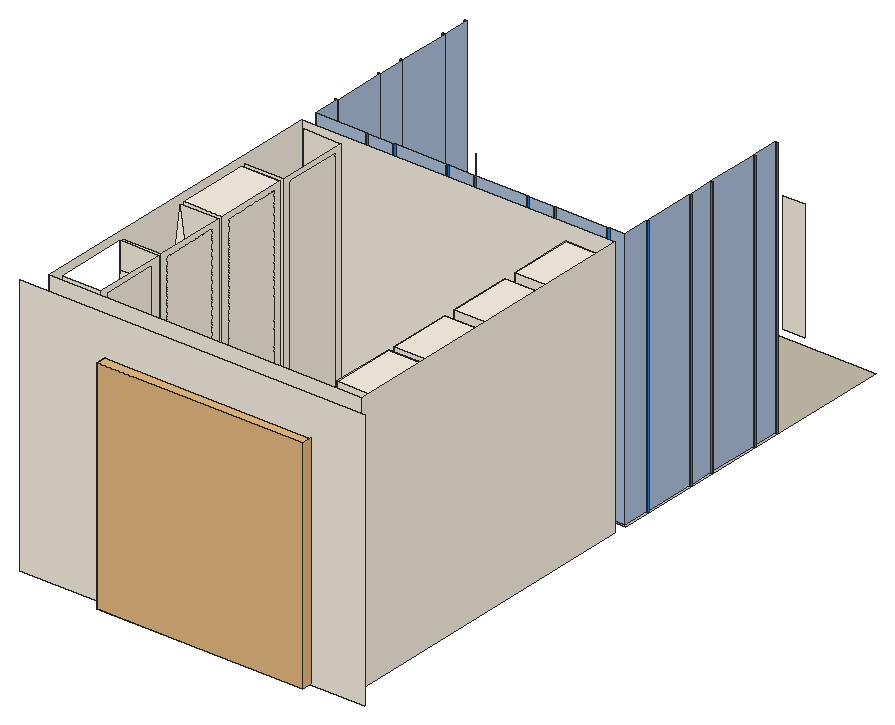
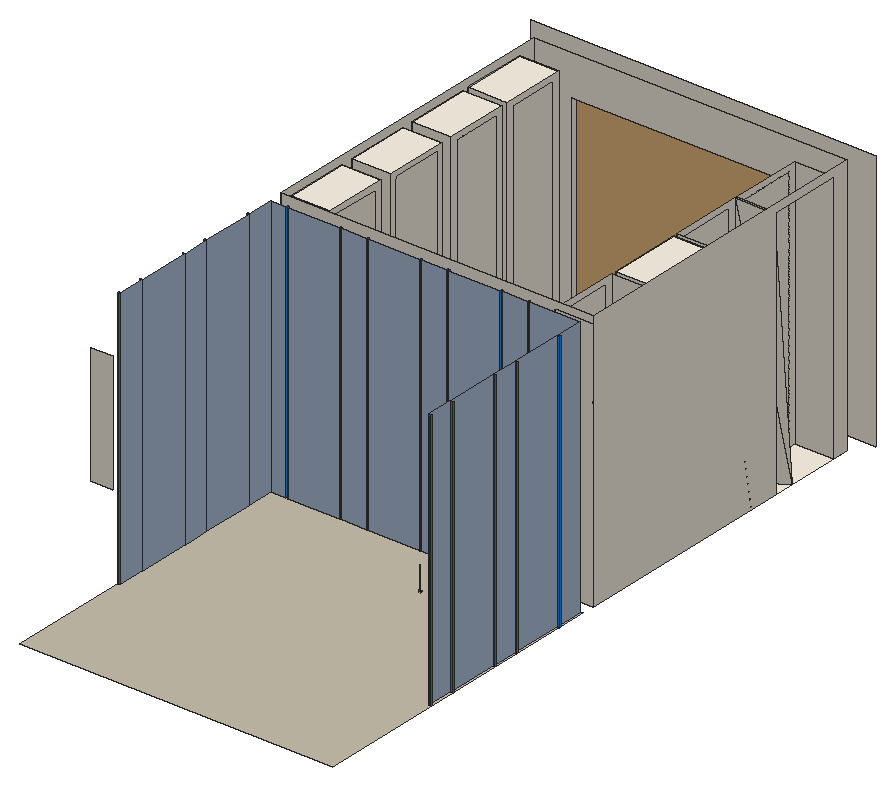
# SketchUp Ruby script. Lengths in inches.
U = 1.inch
M = Sketchup.active_model
def pt(a) = Geom::Point3d.new(a.map { |v| v * U })
def face(e, loops, mat)
  f = e.add_face(loops[0].map { |a| pt(a) })
  loops[1..].each { |l| e.add_face(l.map { |a| pt(a) }).erase! }
  f.material = f.back_material = mat if mat
  f
end
# faces: each face lists its corners as indices into pts; further lists are holes
def faces(e, pts, list, mat = nil) = list.each { |f| face(e, (f[0].is_a?(Array) ? f : [f]).map { |l| l.map { |i| pts[i] } }, mat) }
# xy, xz, yz: faces in a plane at the given z, y or x. An outline is a flat list of corners, or four numbers for a rectangle; further outlines are holes
def ring(l) = l.size == 4 ? [[l[0], l[1]], [l[2], l[1]], [l[2], l[3]], [l[0], l[3]]] : l.each_slice(2).to_a
def flat(e, list, mat, &to3) = list.each { |f| face(e, (f[0].is_a?(Array) ? f : [f]).map { |l| ring(l).map { |u, v| to3.(u, v) } }, mat) }
def xy(e, z, list, mat = nil) = flat(e, list, mat) { |x, y| [x, y, z] }
def xz(e, y, list, mat = nil) = flat(e, list, mat) { |x, z| [x, y, z] }
def yz(e, x, list, mat = nil) = flat(e, list, mat) { |y, z| [x, y, z] }
def lines(e, pts, list) = list.each { |a, b| e.add_line(pt(pts[a]), pt(pts[b])) }
# prism: a flat outline (further loops are holes) pulled along v
def prism(e, loops, v, mat = nil)
  f = face(e, loops, mat); d = Geom::Vector3d.new(v.map { |x| x * U })
  f.pushpull(f.normal.samedirection?(d) ? d.length : -d.length)
end
def box(e, o, s, mat = nil) = prism(e, [[o, [o[0] + s[0], o[1], o[2]], [o[0] + s[0], o[1] + s[1], o[2]], [o[0], o[1] + s[1], o[2]]]], [0, 0, s[2]], mat)
def at(x, y, z, deg = 0) = Geom::Transformation.translation(pt([x, y, z])) * Geom::Transformation.rotation(ORIGIN, Z_AXIS, deg.degrees)
def axes(o, x, y, z) = Geom::Transformation.new([*x, 0, *y, 0, *z, 0, *pt(o).to_a, 1])
def part(name) = M.definitions.add(name)
# library, detail: a bought-in or finely detailed component or shape, given as its bounding box
def library(name, o, s) = part(name).tap { |d| box(d.entities, o, s) }
def detail(e, o, s) = box(e.add_group.entities, o, s)
def put(e, d, t, mat = nil) = e.add_instance(d, t).tap { |i| i.material = mat if mat }
def group(e, t, mat = nil) = e.add_group.tap { |g| g.transformation = t; g.material = mat if mat }.entities
root = M.entities
M.materials.add("Material \#1").color = [140, 140, 140]
M.materials.add("[0030_OldLace]").color = [253, 245, 230]
M.materials.add("[0098_DodgerBlue]").color = [30, 144, 255]
M.materials.add("[0099_LightSteelBlue]").color = [176, 196, 222]
M.materials.add("[Tile Canvas]").color = [199, 192, 173]
c1 = library("Shutters 03 47-19",[-43.47,-3.54,0],[86.94,7.08,66.14])
xy(root,0,[[392.77,22.3125,410.71,51.82],[392.77,54.66,410.71,84.17],[392.77,89.42,410.71,118.93],[392.77,124.42,410.71,153.93]])
xy(root,116.41,[[392.77,22.3125,410.71,51.82],[392.77,54.66,410.71,84.17],[392.77,89.42,410.71,118.93],[267.03,90.88,284.97,124.24],[392.77,124.42,410.71,153.93]],"[0030_OldLace]")
xz(root,4.46,[[261,0,300.25,0,300.25,101.375,393.62,101.375,393.62,0,420,0,420,120,261,120]],"[0030_OldLace]")
xz(root,13.46,[[267,0,267,120,411,120,411,0,393.62,0,393.62,101.375,300.25,101.375,300.25,0]],"[0030_OldLace]")
xz(root,20.99,[[267,0,284.9375,116.41]],"[0030_OldLace]")
xz(root,22.3125,[[392.77,0,410.71,116.41]],"[0030_OldLace]")
xz(root,51.82,[[392.77,0,410.71,116.41]],"[0030_OldLace]")
xz(root,54.35,[[267,0,284.9375,116.41]],"[0030_OldLace]")
xz(root,54.66,[[392.77,0,410.71,116.41]],"[0030_OldLace]")
xz(root,84.17,[[392.77,0,410.71,116.41]],"[0030_OldLace]")
xz(root,88.74,[[284.97,0,267.03,116.41,284.97,116.41]],"[0030_OldLace]")
xz(root,89.42,[[392.77,0,410.71,116.41]],"[0030_OldLace]")
xz(root,90.88,[[267.03,0,284.97,116.41]],"[0030_OldLace]")
xz(root,118.93,[[392.77,0,410.71,116.41]],"[0030_OldLace]")
xz(root,124.24,[[267.03,0,284.97,116.41]],"[0030_OldLace]")
xz(root,124.42,[[392.77,0,410.71,116.41]],"[0030_OldLace]")
xz(root,126.11,[[267.03,0,284.97,116.41]],"[0030_OldLace]")
xz(root,153.93,[[392.77,0,410.71,116.41]],"[0030_OldLace]")
xz(root,159.46,[[267,0,267.03,0,267.03,116.41,284.97,116.41,284.97,0,411,0,411,120,267,120],[267.03,0,284.97,116.41]],"[0030_OldLace]")
xz(root,165.46,[[291.48,0,292.01,120],[304,0,304.5,120],[328.5,0,329,120],[341,0,341.45,120],[365.49,0,366,120],
  [378.01,0,378.5,120],[402.49,0,403,120]],"[0098_DodgerBlue]")
xz(root,166.15,[[267.8125,0,291.48,120],[292.01,0,304,120],[304.5,0,328.5,120],[329,0,341,120],[341.45,0,365.49,120],
  [366,0,378.01,120],[378.5,0,402.49,120],[403,0,410,120]],"[0099_LightSteelBlue]")
xz(root,178.44,[[410,0,411,120]],"[0098_DodgerBlue]")
xz(root,178.47,[[267,0,267.8125,120]],"[0098_DodgerBlue]")
xz(root,178.96,[[267,0,268.125,120]],"[0098_DodgerBlue]")
xz(root,179,[[410,0,411,120]],"[0098_DodgerBlue]")
xz(root,202.96,[[267,0,268.125,120],[410,0,411,120]],"[0098_DodgerBlue]")
xz(root,203.46,[[267,0,268.125,120],[410,0,411,120]],"[0098_DodgerBlue]")
xz(root,215.46,[[267,0,268.125,120],[410,0,411,120]],"[0098_DodgerBlue]")
xz(root,215.96,[[267,0,268.125,120],[410,0,411,120]],"[0098_DodgerBlue]")
xz(root,239.96,[[267,0,268.125,120]],"[0098_DodgerBlue]")
xz(root,239.97,[[410,0,411,120]],"[0098_DodgerBlue]")
xz(root,240.46,[[267,0,268.125,120]],"[0098_DodgerBlue]")
xz(root,240.47,[[410,0,411,120]],"[0098_DodgerBlue]")
xz(root,252.47,[[410,0,411,120]],"[0098_DodgerBlue]")
xz(root,252.53,[[267,0,268.125,120]],"[0098_DodgerBlue]")
xz(root,252.96,[[410,0,411,120]],"[0098_DodgerBlue]")
xz(root,253,[[267,0,268.125,120]],"[0098_DodgerBlue]")
xz(root,257.09,[[410,41,420,96]],"[0030_OldLace]")
yz(root,265.64,[[260.51,50.65,260.4,50.66,260.4,50.68],[260.4,50.66,260.29,50.7,260.29,50.72],[260.4,50.66,260.29,50.72,260.4,50.68],[260.29,50.7,260.18,50.77,260.19,50.78],[260.29,50.7,260.19,50.78,260.29,50.72],
  [260.18,50.77,260.09,50.85,260.1,50.86],[260.18,50.77,260.1,50.86,260.19,50.78],[260.09,50.85,260.02,50.95,260.02,50.96],[260.09,50.85,260.02,50.96,260.1,50.86],[260.48,50.88,260.4375,50.9,260.44,50.91],
  [260.48,50.88,260.44,50.91,260.48,50.9],[260.4375,50.9,260.4,50.92,260.41,50.93],[260.4375,50.9,260.41,50.93,260.44,50.91],[260.4,50.92,260.375,50.95,260.38,50.96],[260.4,50.92,260.38,50.96,260.41,50.93],
  [260.02,50.95,259.96,51.08,260.02,50.96],[260.375,50.95,260.35,50.98,260.36,50.99],[260.375,50.95,260.36,50.99,260.38,50.96],[260.35,50.98,260.33,51.02,260.34,51.03],[260.35,50.98,260.34,51.03,260.36,50.99],
  [260.33,51.02,260.3125,51.07,260.32,51.07],[260.33,51.02,260.32,51.07,260.34,51.03],[260.3125,51.07,260.3,51.12,260.3125,51.12],[260.3125,51.07,260.3125,51.12,260.32,51.07],[260.3,51.12,260.3,51.15,260.31,51.15],
  [260.3,51.12,260.31,51.15,260.3125,51.12],[260.3,51.15,260.3,51.22,260.3125,51.22],[260.3,51.15,260.3125,51.22,260.31,51.15],[260.3,51.22,260.3125,51.27,260.32,51.26],[260.3,51.22,260.32,51.26,260.3125,51.22],
  [260.32,51.26,260.3125,51.27,260.34,51.31],[260.3125,51.27,260.33,51.3125,260.34,51.31],[260.34,51.31,260.33,51.3125,260.36,51.34],[260.33,51.3125,260.35,51.35,260.36,51.34],[260.36,51.34,260.35,51.35,260.38,51.375],
  [260.35,51.35,260.375,51.39,260.38,51.375],[260.38,51.375,260.375,51.39,260.41,51.4],[260.375,51.39,260.4,51.42,260.41,51.4],[260.41,51.4,260.4,51.42,260.44,51.42],[260.4,51.42,260.4375,51.4375,260.44,51.42],
  [260.44,51.42,260.4375,51.4375,260.48,51.4375],[260.4375,51.4375,260.48,51.45,260.48,51.4375]],"Material \#1")
yz(root,266.47,[[260.51,50.65,260.4,50.68,260.4,50.66],[260.4,50.66,260.29,50.72,260.29,50.7],[260.4,50.66,260.4,50.68,260.29,50.72],[260.29,50.7,260.19,50.78,260.18,50.77],[260.29,50.7,260.29,50.72,260.19,50.78],
  [260.18,50.77,260.1,50.86,260.09,50.85],[260.18,50.77,260.19,50.78,260.1,50.86],[260.09,50.85,260.02,50.96,260.02,50.95],[260.09,50.85,260.1,50.86,260.02,50.96],[260.48,50.88,260.44,50.91,260.4375,50.9],
  [260.48,50.88,260.48,50.9,260.44,50.91],[260.4375,50.9,260.41,50.93,260.4,50.92],[260.4375,50.9,260.44,50.91,260.41,50.93],[260.4,50.92,260.38,50.96,260.375,50.95],[260.4,50.92,260.41,50.93,260.38,50.96],
  [260.02,50.95,259.96,51.08,259.95,51.08],[260.02,50.95,260.02,50.96,259.96,51.08],[260.375,50.95,260.36,50.99,260.35,50.98],[260.375,50.95,260.38,50.96,260.36,50.99],[260.35,50.98,260.34,51.03,260.33,51.02],
  [260.35,50.98,260.36,50.99,260.34,51.03],[260.33,51.02,260.32,51.07,260.3125,51.07],[260.33,51.02,260.34,51.03,260.32,51.07],[260.3125,51.07,260.3125,51.12,260.3,51.12],[260.3125,51.07,260.32,51.07,260.3125,51.12],
  [259.95,51.08,259.91,51.22,259.9,51.21],[259.95,51.08,259.96,51.08,259.91,51.22],[260.3,51.12,260.31,51.15,260.3,51.15],[260.3,51.12,260.3125,51.12,260.31,51.15],[260.3,51.15,260.31,51.15,260.3125,51.22],
  [260.3,51.15,260.3125,51.22,260.3,51.22],[259.9,51.21,259.88,51.36,259.87,51.36],[259.9,51.21,259.91,51.22,259.88,51.36],[260.3,51.22,260.3125,51.22,260.32,51.26],[260.3,51.22,260.32,51.26,260.3125,51.27],
  [260.32,51.26,260.34,51.31,260.3125,51.27],[260.3125,51.27,260.34,51.31,260.33,51.3125],[260.34,51.31,260.36,51.34,260.33,51.3125],[260.33,51.3125,260.36,51.34,260.35,51.35],[260.36,51.34,260.38,51.375,260.35,51.35],
  [260.35,51.35,260.38,51.375,260.375,51.39],[259.87,51.36,259.87,51.52,259.86,51.52],[259.87,51.36,259.88,51.36,259.87,51.52],[260.38,51.375,260.41,51.4,260.375,51.39],[260.375,51.39,260.41,51.4,260.4,51.42],
  [260.41,51.4,260.44,51.42,260.4,51.42],[260.4,51.42,260.44,51.42,260.4375,51.4375],[260.44,51.42,260.48,51.4375,260.4375,51.4375],[260.4375,51.4375,260.48,51.4375,260.48,51.45],[259.86,51.52,259.87,51.52,259.87,61.41],
  [259.86,51.52,259.87,61.41,259.86,61.42]],"Material \#1")
yz(root,267,[[13.46,0,20.99,0,20.99,116.41,54.35,116.41,54.35,0,159.46,0,159.46,120,13.46,120]],"[0030_OldLace]")
yz(root,267,[[178.47,0,178.96,120],[202.96,0,203.46,120],[215.46,0,215.96,120],[239.96,0,240.46,120],[252.53,0,253,120]],"[0098_DodgerBlue]")
yz(root,267.8125,[[166.15,0,178.47,120]],"[0099_LightSteelBlue]")
yz(root,268.125,[[178.96,0,202.96,120],[203.46,0,215.46,120],[215.96,0,239.96,120],[240.46,0,252.53,120]],"[0099_LightSteelBlue]")
yz(root,284.9375,[[[20.99,0,54.35,116.41],[24.58,2.54,50.75,113.87]],[24.58,2.54,50.75,113.87]],"[0030_OldLace]")
yz(root,284.97,[[[55.39,0,88.74,116.41],[58.98,2.54,85.15,113.87]],[[90.88,0,124.24,116.41],[94.47,2.54,120.64,113.87]],[[126.11,0,159.46,116.41],[129.7,2.54,155.875,113.87]],[58.98,2.54,85.15,113.87],[94.47,2.54,120.64,113.87],
  [129.7,2.54,155.875,113.87]],"[0030_OldLace]")
yz(root,291.48,[[165.46,0,166.15,120]],"[0098_DodgerBlue]")
yz(root,292.01,[[165.46,0,166.15,120]],"[0098_DodgerBlue]")
yz(root,300.25,[[4.46,0,13.46,101.375]],"[0030_OldLace]")
yz(root,304,[[165.46,0,166.15,120]],"[0098_DodgerBlue]")
yz(root,304.5,[[165.46,0,166.15,120]],"[0098_DodgerBlue]")
yz(root,328.5,[[165.46,0,166.15,120]],"[0098_DodgerBlue]")
yz(root,329,[[165.46,0,166.15,120]],"[0098_DodgerBlue]")
yz(root,341,[[165.46,0,166.15,120]],"[0098_DodgerBlue]")
yz(root,341.45,[[165.46,0,166.15,120]],"[0098_DodgerBlue]")
yz(root,365.49,[[165.46,0,166.15,120]],"[0098_DodgerBlue]")
yz(root,366,[[165.46,0,166.15,120]],"[0098_DodgerBlue]")
yz(root,378.01,[[165.46,0,166.15,120]],"[0098_DodgerBlue]")
yz(root,378.5,[[165.46,0,166.15,120]],"[0098_DodgerBlue]")
yz(root,392.77,[[[22.3125,0,51.82,116.41],[25.49,2.54,48.65,113.87]],[[54.66,0,84.17,116.41],[57.83,2.54,80.99,113.87]],[[89.42,0,118.93,116.41],[92.6,2.54,115.76,113.87]],[[124.42,0,153.93,116.41],[127.6,2.54,150.76,113.87]],[25.49,2.54,48.65,113.87],
  [57.83,2.54,80.99,113.87],[92.6,2.54,115.76,113.87],[127.6,2.54,150.76,113.87]],"[0030_OldLace]")
yz(root,393.62,[[4.46,0,13.46,101.375]],"[0030_OldLace]")
yz(root,402.49,[[165.46,0,166.15,120]],"[0098_DodgerBlue]")
yz(root,403,[[165.46,0,166.15,120]],"[0098_DodgerBlue]")
yz(root,410,[[166.15,0,178.44,120],[179,0,202.96,120],[203.46,0,215.46,120],[215.96,0,239.97,120],[240.47,0,252.47,120]],"[0099_LightSteelBlue]")
yz(root,410.71,[[22.3125,0,51.82,116.41],[54.66,0,84.17,116.41],[89.42,0,118.93,116.41],[124.42,0,153.93,116.41]])
yz(root,411,[[13.46,0,159.46,120]],"[0030_OldLace]")
yz(root,411,[[178.44,0,179,120],[202.96,0,203.46,120],[215.46,0,215.96,120],[239.97,0,240.47,120],[252.47,0,252.96,120]],"[0098_DodgerBlue]")
p = [[267.03,55.39,116.41],[267.03,45.34,0],[284.97,55.39,116.41],[284.97,55.39,0],[283.11,54.35,0],[267.03,68.95,0],
  [267.03,88.74,116.41],[284.97,88.74,0],[300.25,13.46,0],[393.62,13.46,0]]
faces(root,p,[[0,1,2],[3,2,1,4],[5,6,7]],"[0030_OldLace]")
lines(root,p,[[8,9]])
put(root,c1,axes([347.45,5.78,0],[1.09,0,0],[0,1.63,0],[0,0,1.53268]))
g1 = group(root,at(267,13.46,0),"[0030_OldLace]")
xy(g1,0,[[0,0,144,146]])
g2 = group(root,at(267,165.46,0),"[Tile Canvas]")
xy(g2,0,[[0,0,144,144]])
